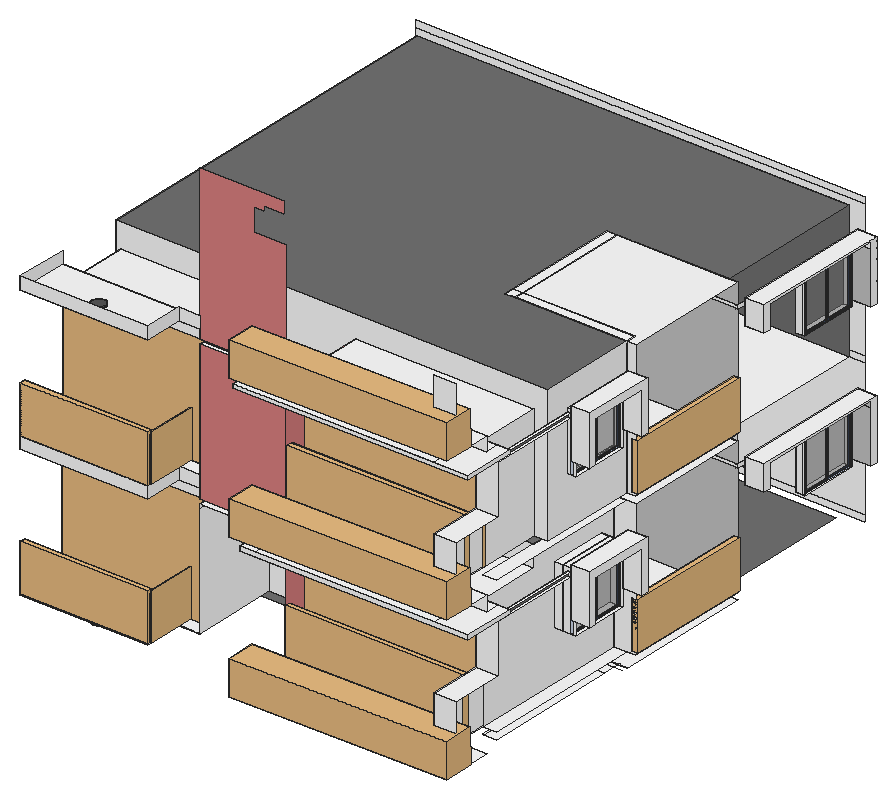
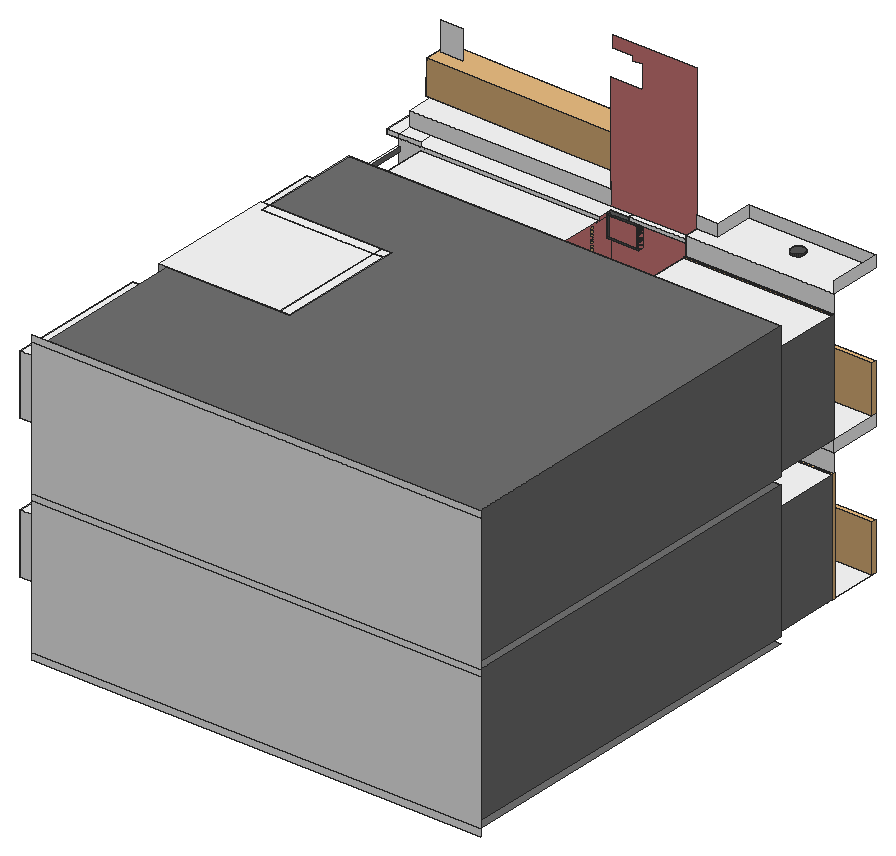
# SketchUp Ruby script. Lengths in inches.
U = 1.inch
M = Sketchup.active_model
def pt(a) = Geom::Point3d.new(a.map { |v| v * U })
def face(e, loops, mat)
  f = e.add_face(loops[0].map { |a| pt(a) })
  loops[1..].each { |l| e.add_face(l.map { |a| pt(a) }).erase! }
  f.material = f.back_material = mat if mat
  f
end
# faces: each face lists its corners as indices into pts; further lists are holes
def faces(e, pts, list, mat = nil) = list.each { |f| face(e, (f[0].is_a?(Array) ? f : [f]).map { |l| l.map { |i| pts[i] } }, mat) }
# xy, xz, yz: faces in a plane at the given z, y or x. An outline is a flat list of corners, or four numbers for a rectangle; further outlines are holes
def ring(l) = l.size == 4 ? [[l[0], l[1]], [l[2], l[1]], [l[2], l[3]], [l[0], l[3]]] : l.each_slice(2).to_a
def flat(e, list, mat, &to3) = list.each { |f| face(e, (f[0].is_a?(Array) ? f : [f]).map { |l| ring(l).map { |u, v| to3.(u, v) } }, mat) }
def xy(e, z, list, mat = nil) = flat(e, list, mat) { |x, y| [x, y, z] }
def xz(e, y, list, mat = nil) = flat(e, list, mat) { |x, z| [x, y, z] }
def yz(e, x, list, mat = nil) = flat(e, list, mat) { |y, z| [x, y, z] }
def lines(e, pts, list) = list.each { |a, b| e.add_line(pt(pts[a]), pt(pts[b])) }
# prism: a flat outline (further loops are holes) pulled along v
def prism(e, loops, v, mat = nil)
  f = face(e, loops, mat); d = Geom::Vector3d.new(v.map { |x| x * U })
  f.pushpull(f.normal.samedirection?(d) ? d.length : -d.length)
end
def box(e, o, s, mat = nil) = prism(e, [[o, [o[0] + s[0], o[1], o[2]], [o[0] + s[0], o[1] + s[1], o[2]], [o[0], o[1] + s[1], o[2]]]], [0, 0, s[2]], mat)
def at(x, y, z, deg = 0) = Geom::Transformation.translation(pt([x, y, z])) * Geom::Transformation.rotation(ORIGIN, Z_AXIS, deg.degrees)
def axes(o, x, y, z) = Geom::Transformation.new([*x, 0, *y, 0, *z, 0, *pt(o).to_a, 1])
def part(name) = M.definitions.add(name)
# library, detail: a bought-in or finely detailed component or shape, given as its bounding box
def library(name, o, s) = part(name).tap { |d| box(d.entities, o, s) }
def detail(e, o, s) = box(e.add_group.entities, o, s)
def put(e, d, t, mat = nil) = e.add_instance(d, t).tap { |i| i.material = mat if mat }
def group(e, t, mat = nil) = e.add_group.tap { |g| g.transformation = t; g.material = mat if mat }.entities
root = M.entities
M.materials.add("[Color M00]").color = [255, 255, 255]
M.materials.add("[Color M02]").color = [198, 198, 198]
M.materials.add("[Color M05]").color = [114, 114, 114]
M.materials.add("[Color M06]").color = [86, 86, 86]
M.materials.add("[Color_006]").color = [86, 86, 86]
M.materials.add("[Tile Various Tan]").color = [221, 130, 130]
M.materials.add("[Translucent Glass Blue]").color = [74, 111, 178]
M.materials["[Translucent Glass Blue]"].alpha = 0.26
M.materials.add("[Translucent Glass Gray]").color = [128, 128, 128]
M.materials["[Translucent Glass Gray]"].alpha = 0.5
M.materials.add("[Translucent_Glass_Gray]").color = [167, 187, 214]
M.materials["[Translucent_Glass_Gray]"].alpha = 0.8
c1 = library("Living wall panel",[-0.54,-4.26,-5.13],[55.52,26.12,125.59])
c2 = library("Glass Railing",[0,0,0],[139.5,4.76,42])
c3 = library("Glazed balcony doors",[0,0,0],[135.86,2.83,115.35])
c4 = part("glass-railing")
detail(c4.entities,[0,0,0],[1.26,75.59,33.1875])
c5 = part("Group\#3")
xy(c5.entities,0,[[0,0,32.48,1.97]])
xy(c5.entities,0.98,[[0.98,0,31.5,0.98],[0.98,0.98,31.5,1.97]])
xy(c5.entities,8.86,[[0.98,0,31.5,0.98],[0.98,0.98,31.5,1.97]])
xy(c5.entities,9.84,[[0,0,32.48,1.97]])
xz(c5.entities,0,[[[0,0,32.48,9.84],[0.98,0.98,31.5,8.86]]])
xz(c5.entities,0.98,[[0.98,0.98,31.5,8.86]],"[Translucent Glass Gray]")
xz(c5.entities,1.97,[[[0,0,32.48,9.84],[0.98,0.98,31.5,8.86]]])
yz(c5.entities,0,[[0,0,1.97,9.84]])
yz(c5.entities,0.98,[[0,0.98,0.98,8.86],[0.98,0.98,1.97,8.86]])
yz(c5.entities,31.5,[[0,0.98,0.98,8.86],[0.98,0.98,1.97,8.86]])
yz(c5.entities,32.48,[[0,0,1.97,9.84]])
c6 = part("Group\#4")
xy(c6.entities,0,[[0,0,32.48,1.97]])
xy(c6.entities,0.98,[[0.98,0,31.5,0.98],[0.98,0.98,31.5,1.97]])
xy(c6.entities,71.85,[[0.98,0,31.5,0.98],[0.98,0.98,31.5,1.97]])
xy(c6.entities,72.83,[[0,0,32.48,1.97]])
xz(c6.entities,0,[[[0,0,32.48,72.83],[0.98,0.98,31.5,71.85]]])
xz(c6.entities,0.98,[[0.98,0.98,31.5,71.85]],"[Translucent Glass Gray]")
xz(c6.entities,1.97,[[[0,0,32.48,72.83],[0.98,0.98,31.5,71.85]]])
yz(c6.entities,0,[[0,0,1.97,72.83]])
yz(c6.entities,0.98,[[0,0.98,0.98,71.85],[0.98,0.98,1.97,71.85]])
yz(c6.entities,31.5,[[0,0.98,0.98,71.85],[0.98,0.98,1.97,71.85]])
yz(c6.entities,32.48,[[0,0,1.97,72.83]])
c7 = part("Fixed transom window")
xy(c7.entities,0,[[0,0,70.86,3.9375]])
xy(c7.entities,1.97,[[1.97,0,34.45,0.98],[36.42,0,68.9,3.9375],[1.97,2.95,34.45,3.9375]])
xy(c7.entities,86.61,[[1.97,0,34.45,3.9375],[34.45,0,36.42,3.9375],[36.42,0,68.9,3.9375]])
xy(c7.entities,88.58,[[0,0,70.86,3.9375]])
xz(c7.entities,0,[[[0,0,70.86,88.58],[1.97,1.97,34.45,86.61],[36.42,1.97,68.9,86.61]]])
xz(c7.entities,3.9375,[[[0,0,70.86,88.58],[1.97,1.97,34.45,86.61],[36.42,1.97,68.9,86.61]]])
yz(c7.entities,0,[[0,0,3.9375,88.58]])
yz(c7.entities,1.97,[[0,1.97,3.9375,74.8],[0,76.77,3.9375,86.61]])
yz(c7.entities,34.45,[[0,1.97,3.9375,86.61]])
yz(c7.entities,36.42,[[0,1.97,3.9375,86.61]])
yz(c7.entities,68.9,[[0,1.97,3.9375,86.61]])
yz(c7.entities,70.86,[[0,0,3.9375,88.58]])
g1 = group(c7.entities,at(1.97,0,74.8))
box(g1,[0,0,0],[66.93,3.9375,1.97])
put(c7.entities,c5,at(1.97,0.98,76.77),"[Translucent Glass Blue]")
put(c7.entities,c5,at(36.42,0.98,76.77),"[Translucent Glass Blue]")
put(c7.entities,c6,at(1.97,0.98,1.97),"[Translucent Glass Blue]")
put(c7.entities,c6,at(36.42,0.98,1.97),"[Translucent Glass Blue]")
c8 = part("FIXED+GLASS+WINDOW+WITH+TRANSOM")
put(c8.entities,c7,at(0,0,0),"[Translucent Glass Blue]")
c9 = part("BIC_Bike Shop - Window - Small")
xy(c9.entities,-8,[[[0,0,36,36],[2,2,34,34]]],"[Color_006]")
xy(c9.entities,-4,[[2,2,34,34]],"[Translucent_Glass_Gray]")
xy(c9.entities,0,[[[0,0,36,36],[2,2,34,34]]],"[Color_006]")
xz(c9.entities,0,[[0,-8,36,0]],"[Color_006]")
xz(c9.entities,2,[[2,-8,34,-4],[2,-4,34,0]],"[Color_006]")
xz(c9.entities,34,[[2,-8,34,-4],[2,-4,34,0]],"[Color_006]")
xz(c9.entities,36,[[0,-8,36,0]],"[Color_006]")
yz(c9.entities,0,[[0,-8,36,0]],"[Color_006]")
yz(c9.entities,2,[[2,-8,34,-4],[2,-4,34,0]],"[Color_006]")
yz(c9.entities,34,[[2,-8,34,-4],[2,-4,34,0]],"[Color_006]")
yz(c9.entities,36,[[0,-8,36,0]],"[Color_006]")
xy(root,374.8125,[[129.49,93.91,127.93,94.12,126.49,94.72,125.24,95.67,124.29,96.91,123.69,98.36,123.49,99.91,123.69,101.46,124.29,102.91,125.24,104.15,126.49,105.11,127.93,105.71,129.49,105.91,131.04,105.71,132.49,105.11,133.73,104.15,134.68,102.91,135.28,101.46,135.49,99.91,135.28,98.36,134.68,96.91,133.73,95.67,132.49,94.72,131.04,94.12]],"[Color M06]")
xy(root,377.5625,[[281.18,83.25,458.625,117.625],[439.42,137.58,439.8125,257.51],[439.8125,137.58,450.92,257.51],[330.6875,194.2,330.6875,281.78,385.6875,281.78,385.6875,273.63,401.8125,273.63,401.8125,257.51,439.42,257.51,439.42,194.2],[401.8125,257.51,439.42,267.63],
  [439.42,257.51,450.92,267.63],[401.8125,267.63,439.42,272.07],[439.42,267.63,450.92,272.07],[401.8125,272.07,439.42,273.63],[439.42,272.07,450.92,273.63],
  [450.92,272.07,458.625,273.63],[385.6875,273.63,401.8125,281.78],[401.8125,273.63,458.625,394.46],[385.6875,281.78,401.8125,394.46]],"[Color M00]")
xy(root,377.5625,[[69.2,194.2,69.2,527.42,439.42,527.42,439.42,394.46,385.6875,394.46,385.6875,281.78,330.6875,281.78,330.6875,194.2]],"[Color M05]")
xy(root,383.5625,[[73.74,83.25,73.74,137.58,204.98,137.58,204.98,117.625,186.35,117.625,186.35,83.25],[281.18,91.3,439.11,137.58],[73.74,137.58,204.98,137.58,204.98,194.2,281.18,194.2,281.18,137.58,439.11,137.58,439.11,281.78,351.1875,281.78,351.1875,527.42,69.2,527.42,69.2,194.2,73.74,194.2],[439.11,137.58,450.92,281.78],[351.1875,281.78,439.11,290.48],
  [439.11,281.78,450.92,281.78,450.92,394.46,351.1875,394.46,351.1875,290.48,439.11,290.48],[450.92,281.78,458.625,394.46]],"[Color M00]")
xy(root,383.8125,[[73.74,83.25,186.35,83.25,186.35,117.625,204.98,117.625,204.98,137.58,73.74,137.58],[281.18,91.3,439.11,137.58]],"[Color M00]")
xy(root,397,[[281.18,83.25,439.11,91.3]],"[Color M00]")
xy(root,397.25,[[281.18,83.25,439.11,91.3]],"[Color M00]")
xy(root,427.98,[[438.17,215.57,446.875,267.63],[446.875,215.57,458.625,267.63],[450.92,468.92,458.625,520.98]],"[Color M00]")
xy(root,433.84,[[439.11,83.25,458.625,129.875]],"[Color M00]")
xy(root,434.24,[[458.625,520.98,475.1875,526.98]],"[Color M00]")
xy(root,442.95,[[458.625,210.07,475.5625,215.57],[458.625,267.63,475.5625,273.63]],"[Color M00]")
xy(root,465.36,[[458.625,402.98,475.1875,408.98]],"[Color M00]")
xy(root,466.54,[[252.64,117.625,281.18,122.0625]],"[Tile Various Tan]")
xy(root,477.21,[[456.375,130.82,458.625,210.07]],"[Color M00]")
xy(root,480.05,[[438.17,215.57,446.875,267.63],[446.875,215.57,458.625,267.63],[458.625,215.57,475.5625,267.63],[450.92,468.92,458.625,520.98]],"[Color M00]")
xy(root,481.21,[[456.375,130.82,458.625,210.07]],"[Color M00]")
xy(root,482.19,[[381.625,394.46,385.6875,394.83],[385.6875,394.46,401.8125,394.83],[401.8125,394.46,458.625,394.83]],"[Color M00]")
xy(root,482.48,[[73.74,129.875,204.98,194.2]],"[Color M00]")
xy(root,484.125,[[281.18,129.875,439.11,194.2]],"[Color M00]")
xy(root,485.48,[[381.625,394.46,385.6875,394.83],[385.6875,394.46,401.8125,394.83],[401.8125,394.46,458.625,394.83],[458.625,394.46,459,400.46]],"[Color M00]")
xy(root,485.49,[[458.625,408.98,475.1875,520.98]],"[Color M00]")
xy(root,486.52,[[267.54,83.25,267.54,122.0625,281.18,122.0625,281.18,129.875,468.99,129.875,468.99,83.25],[204.98,117.625,252.64,117.625,252.64,122.0625,267.54,122.0625,267.54,123.3125,204.98,123.3125]],"[Color M00]")
xy(root,486.64,[[458.625,210.07,475.5625,273.63]],"[Color M00]")
xy(root,487.3,[[458.625,402.98,475.1875,526.98]],"[Color M00]")
xy(root,490.2,[[267.54,83.25,281.18,117.625],[281.18,83.25,439.24,117.625],[439.24,83.25,468.99,83.25,468.99,129.875,458.625,129.875,458.625,117.625,439.24,117.625],[204.98,117.625,267.54,123.3125],[439.24,117.625,458.625,129.875]],"[Color M00]")
xy(root,498.9375,[[[73.74,83.25,73.74,129.875,204.98,129.875,204.98,117.625,186.35,117.625,186.35,83.25],[129.49,93.91,131.04,94.12,132.49,94.72,133.73,95.67,134.68,96.91,135.28,98.36,135.49,99.91,135.28,101.46,134.68,102.91,133.73,104.15,132.49,105.11,131.04,105.71,129.49,105.91,127.93,105.71,126.49,105.11,125.24,104.15,124.29,102.91,123.69,101.46,123.49,99.91,123.69,98.36,124.29,96.91,125.24,95.67,126.49,94.72,127.93,94.12]]],"[Color M00]")
xy(root,500.8125,[[129.49,93.91,127.93,94.12,126.49,94.72,125.24,95.67,124.29,96.91,123.69,98.36,123.49,99.91,123.69,101.46,124.29,102.91,125.24,104.15,126.49,105.11,127.93,105.71,129.49,105.91,131.04,105.71,132.49,105.11,133.73,104.15,134.68,102.91,135.28,101.46,135.49,99.91,135.28,98.36,134.68,96.91,133.73,95.67,132.49,94.72,131.04,94.12]],"[Color M06]")
xy(root,503.5625,[[281.18,83.25,458.625,117.625],[439.11,137.58,450.92,281.78],[351.1875,281.78,439.11,290.48],[439.11,281.78,439.11,290.48,351.1875,290.48,351.1875,394.46,458.625,394.46,458.625,281.78]],"[Color M00]")
xy(root,503.5625,[[69.2,194.2,69.2,527.42,351.1875,527.42,351.1875,281.78,439.11,281.78,439.11,194.2]],"[Color M05]")
xy(root,509.5625,[[73.74,83.25,186.35,83.25,186.35,117.625,204.98,117.625,204.98,129.875,73.74,129.875],[281.18,91.3,439.11,137.58],[73.74,129.875,204.98,137.58],[73.74,137.58,204.98,137.58,204.98,194.2,281.18,194.2,281.18,137.58,343.48,137.58,343.48,394.46,450.92,394.46,450.92,527.42,69.2,527.42,69.2,194.2,73.74,194.2],[343.48,137.58,439.11,137.58,439.11,194.2,450.92,194.2,450.92,281.78,343.48,281.78],
  [343.48,281.78,352.1875,290.48],[352.1875,281.78,450.92,290.48],[450.92,281.78,458.625,394.46],[343.48,290.48,352.1875,394.46],[352.1875,290.48,450.92,394.46]],"[Color M00]")
xy(root,509.8125,[[281.18,91.3,439.11,137.58],[73.74,129.875,204.98,137.58]],"[Color M00]")
xy(root,523,[[281.18,83.25,439.11,91.3]],"[Color M00]")
xy(root,523.25,[[281.18,83.25,439.11,91.3]],"[Color M00]")
xy(root,553.98,[[450.92,215.57,458.625,267.63],[450.92,468.92,458.625,520.98]],"[Color M00]")
xy(root,559.84,[[439.11,83.25,458.625,129.875]],"[Color M00]")
xy(root,560.24,[[458.625,520.98,475.1875,526.98]],"[Color M00]")
xy(root,568.95,[[458.625,210.07,475.5625,215.57],[458.625,267.63,475.5625,273.63]],"[Color M00]")
xy(root,591.36,[[458.625,402.98,475.1875,408.98]],"[Color M00]")
xy(root,592.97,[[252.64,117.625,281.18,121.75]],"[Tile Various Tan]")
xy(root,603.27,[[456.375,130.82,458.625,210.07]],"[Color M00]")
xy(root,606.05,[[450.92,215.57,458.625,267.63],[458.625,215.57,475.5625,267.63],[450.92,468.92,458.625,520.98]],"[Color M00]")
xy(root,607.27,[[456.375,130.82,458.625,210.07]],"[Color M00]")
xy(root,608.19,[[381.625,394.46,385.6875,394.83],[385.6875,394.46,401.8125,394.83],[401.8125,394.46,458.625,394.83]],"[Color M00]")
xy(root,608.48,[[73.74,129.875,204.98,194.2]],"[Color M00]")
xy(root,610.125,[[281.18,129.875,439.11,194.2]],"[Color M00]")
xy(root,611.48,[[381.625,394.46,385.6875,394.83],[385.6875,394.46,401.8125,394.83],[401.8125,394.46,458.625,394.83],[458.625,394.46,459,400.46]],"[Color M00]")
xy(root,611.49,[[458.625,408.98,475.1875,520.98]],"[Color M00]")
xy(root,612.64,[[458.625,210.07,475.5625,273.63]],"[Color M00]")
xy(root,612.95,[[261.54,83.25,261.54,121.75,281.18,121.75,281.18,129.875,468.99,129.875,468.99,83.25],[204.98,117.625,252.64,121.75]],"[Color M00]")
xy(root,613.3,[[458.625,402.98,475.1875,526.98]],"[Color M00]")
xy(root,616.64,[[261.54,83.25,439.24,117.625],[439.24,83.25,468.99,83.25,468.99,129.875,458.625,129.875,458.625,117.625,439.24,117.625],[204.98,117.625,261.54,121.75],[439.24,117.625,458.625,129.875]],"[Color M00]")
xy(root,624.9375,[[[73.74,83.25,73.74,129.875,204.98,129.875,204.98,117.625,186.35,117.625,186.35,83.25],[129.49,93.91,131.04,94.12,132.49,94.72,133.73,95.67,134.68,96.91,135.28,98.36,135.49,99.91,135.28,101.46,134.68,102.91,133.73,104.15,132.49,105.11,131.04,105.71,129.49,105.91,127.93,105.71,126.49,105.11,125.24,104.15,124.29,102.91,123.69,101.46,123.49,99.91,123.69,98.36,124.29,96.91,125.24,95.67,126.49,94.72,127.93,94.12]]],"[Color M00]")
xy(root,626.8125,[[129.49,93.91,127.93,94.12,126.49,94.72,125.24,95.67,124.29,96.91,123.69,98.36,123.49,99.91,123.69,101.46,124.29,102.91,125.24,104.15,126.49,105.11,127.93,105.71,129.49,105.91,131.04,105.71,132.49,105.11,133.73,104.15,134.68,102.91,135.28,101.46,135.49,99.91,135.28,98.36,134.68,96.91,133.73,95.67,132.49,94.72,131.04,94.12]],"[Color M06]")
xy(root,629.5625,[[281.18,83.25,458.625,117.625],[343.48,281.78,352.1875,290.48],[352.1875,281.78,450.92,290.48],[450.92,281.78,450.92,290.48,352.1875,290.48,352.1875,394.46,458.625,394.46,458.625,281.78],[343.48,290.48,352.1875,394.46]],"[Color M00]")
xy(root,629.5625,[[69.2,194.2,69.2,527.42,450.92,527.42,450.92,394.46,343.48,394.46,343.48,281.78,450.92,281.78,450.92,194.2]],"[Color M05]")
xz(root,83.25,[[281.18,377.5625,458.625,377.5625,458.625,433.84,439.11,433.84,439.11,397,281.18,397],[73.74,383.5625,186.35,383.8125],[281.18,397,439.11,397.25],[267.54,486.52,468.99,490.2],[73.74,498.9375,186.35,509.5625],
  [281.18,503.5625,458.625,503.5625,458.625,559.84,439.11,559.84,439.11,523,281.18,523],[281.18,523,439.11,523.25],[261.54,612.95,468.99,616.64],[73.74,624.9375,186.35,635.5625],[281.18,629.5625,458.625,629.5625,458.625,685.84,439.11,685.84,439.11,649,281.18,649]],"[Color M00]")
xz(root,91.3,[[281.18,383.5625,439.11,383.8125],[281.18,383.8125,439.11,397],[281.18,397,439.11,397.25],[281.18,509.5625,439.11,509.8125],[281.18,509.8125,439.11,523],
  [281.18,523,439.11,523.25]],"[Color M00]")
xz(root,117.625,[[186.35,383.5625,204.98,383.8125],[281.18,490.2,458.625,503.5625],[186.35,498.9375,204.98,509.5625],[281.18,616.64,458.625,629.5625],[186.35,624.9375,204.98,635.5625]],"[Color M00]")
xz(root,117.625,[[204.98,490.2,281.18,490.2,281.18,592.97,252.64,592.97,252.64,612.95,204.98,612.95],[204.98,616.64,281.18,616.64,281.18,718.41,252.64,718.41,252.64,738.39,261.54,738.39,261.54,742.08,279.24,742.08,279.24,752.39,204.98,752.39]],"[Tile Various Tan]")
xz(root,121.75,[[204.98,612.95,261.54,616.64]],"[Color M00]")
xz(root,121.75,[[252.64,592.97,281.18,612.95]],"[Tile Various Tan]")
xz(root,122.0625,[[252.64,466.54,281.18,486.52]],"[Tile Various Tan]")
xz(root,123.3125,[[204.98,486.52,267.54,490.2]],"[Color M00]")
xz(root,129.875,[[439.11,433.84,458.625,433.84,458.625,486.52,281.18,486.52,281.18,484.125,439.11,484.125],[73.74,482.48,204.98,498.9375],[439.24,486.52,458.625,490.2],[458.625,486.52,468.99,490.2],[73.74,498.9375,204.98,509.5625],
  [73.74,509.5625,204.98,509.8125],[439.11,559.84,458.625,559.84,458.625,612.95,281.18,612.95,281.18,610.125,439.11,610.125],[73.74,608.48,204.98,624.9375],[439.24,612.95,458.625,616.64],[458.625,612.95,468.99,616.64]],"[Color M00]")
xz(root,130.82,[[456.375,477.21,458.625,481.21],[456.375,603.27,458.625,607.27]],"[Color M00]")
xz(root,137.58,[[73.74,383.5625,204.98,383.8125],[281.18,383.5625,439.11,383.8125],[73.74,509.5625,204.98,509.8125],[281.18,509.5625,343.48,509.8125],[343.48,509.5625,439.11,509.8125]],"[Color M00]")
xz(root,194.2,[[69.2,383.5625,69.2,503.5625,439.11,503.5625,439.11,484.125,281.18,484.125,281.18,383.5625,204.98,383.5625,204.98,482.48,73.74,482.48,73.74,383.5625],[69.2,509.5625,69.2,629.5625,450.92,629.5625,450.92,509.5625,439.11,509.5625,439.11,610.125,281.18,610.125,281.18,509.5625,204.98,509.5625,204.98,608.48,73.74,608.48,73.74,509.5625]],"[Color M00]")
xz(root,210.07,[[458.625,442.95,475.5625,486.64],[456.375,477.21,458.625,480.05],[456.375,480.05,458.625,481.21],[458.625,568.95,475.5625,612.64],[456.375,603.27,458.625,606.11],
  [456.375,606.11,458.625,607.27]],"[Color M00]")
xz(root,215.57,[[438.17,427.98,446.875,480.05],[446.875,427.98,458.625,480.05],[458.625,442.95,475.5625,480.05],[450.92,553.98,458.625,606.05],[458.625,568.95,475.5625,606.05]],"[Color M00]")
xz(root,267.63,[[438.17,427.98,446.875,480.05],[446.875,427.98,458.625,480.05],[458.625,442.95,475.5625,480.05],[450.92,553.98,458.625,606.05],[458.625,568.95,475.5625,606.05]],"[Color M00]")
xz(root,273.63,[[458.625,442.95,475.5625,486.64],[458.625,568.95,475.5625,612.64]],"[Color M00]")
xz(root,281.78,[[351.1875,383.5625,439.11,503.5625],[439.11,383.5625,458.625,503.5625],[343.48,509.5625,352.1875,629.5625],[352.1875,509.5625,450.92,629.5625],[450.92,509.5625,458.625,629.5625]],"[Color M00]")
xz(root,290.48,[[351.1875,383.5625,439.11,503.5625],[343.48,509.5625,352.1875,629.5625],[352.1875,509.5625,450.92,629.5625]],"[Color M00]")
xz(root,394.46,[[343.48,509.5625,352.1875,629.5625]],"[Color M00]")
xz(root,394.46,[[351.1875,383.5625,458.625,383.5625,458.625,482.19,381.625,482.19,381.625,485.48,458.625,485.48,458.625,503.5625,351.1875,503.5625],[352.1875,509.5625,458.625,509.5625,458.625,608.19,381.625,608.19,381.625,611.48,458.625,611.48,458.625,629.5625,352.1875,629.5625]],"[Color M02]")
xz(root,394.83,[[381.625,482.19,458.625,485.48],[381.625,608.19,458.625,611.48]],"[Color M00]")
xz(root,400.46,[[458.625,482.11,459,485.48],[458.625,608.11,459,611.48]],"[Color M00]")
xz(root,402.98,[[458.625,465.36,475.1875,487.3],[458.625,591.36,475.1875,613.3]],"[Color M00]")
xz(root,408.98,[[458.625,465.36,475.1875,479.49],[458.625,479.49,475.1875,485.49],[458.625,591.36,475.1875,605.49],[458.625,605.49,475.1875,611.49]],"[Color M00]")
xz(root,468.92,[[450.92,427.98,458.625,480.05],[450.92,553.98,458.625,606.05]],"[Color M00]")
xz(root,520.98,[[450.92,427.98,458.625,480.05],[450.92,553.98,458.625,606.05],[458.625,606.05,475.1875,611.49]],"[Color M00]")
xz(root,520.98,[[458.625,434.24,475.1875,480.05],[458.625,480.05,475.1875,485.49],[458.625,560.24,475.1875,606.05]],"[Color M02]")
xz(root,526.98,[[458.625,434.24,475.1875,487.3],[458.625,560.24,475.1875,613.3]],"[Color M00]")
xz(root,527.42,[[69.2,383.5625,351.1875,503.5625],[69.2,509.5625,450.92,629.5625]],"[Color M05]")
xz(root,535.125,[[61.5,377.5625,458.625,383.5625],[61.5,383.5625,458.625,503.5625],[61.5,503.5625,458.625,509.5625],[61.5,509.5625,458.625,629.5625],[61.5,629.5625,458.625,635.5625]],"[Color M00]")
yz(root,69.2,[[194.2,383.5625,527.42,503.5625],[194.2,509.5625,527.42,629.5625]],"[Color M05]")
yz(root,73.74,[[83.25,383.5625,129.875,383.8125],[129.875,383.5625,137.58,383.8125],[83.25,498.9375,129.875,509.5625],[129.875,509.5625,137.58,509.8125],[83.25,624.9375,129.875,635.5625]],"[Color M00]")
yz(root,73.74,[[137.58,383.5625,194.2,383.5625,194.2,482.48,129.875,482.48,129.875,383.8125,137.58,383.8125],[137.58,509.5625,194.2,509.5625,194.2,608.48,129.875,608.48,129.875,509.8125,137.58,509.8125]],"[Color M05]")
yz(root,186.35,[[83.25,383.5625,117.625,383.8125],[83.25,498.9375,117.625,509.5625],[83.25,624.9375,117.625,635.5625]],"[Color M00]")
yz(root,204.98,[[117.625,383.5625,137.58,383.8125],[137.58,383.5625,137.58,383.8125,117.625,383.8125,117.625,482.48,194.2,482.48,194.2,383.5625],[117.625,482.48,117.625,486.52,123.3125,486.52,123.3125,490.2,117.625,490.2,117.625,498.9375,129.875,498.9375,129.875,482.48],[117.625,498.9375,129.875,509.5625],[117.625,509.5625,117.625,608.48,194.2,608.48,194.2,509.5625,137.58,509.5625,137.58,509.8125,129.875,509.8125,129.875,509.5625],
  [129.875,509.5625,137.58,509.8125],[117.625,608.48,117.625,612.95,121.75,612.95,121.75,616.64,117.625,616.64,117.625,624.9375,129.875,624.9375,129.875,608.48]],"[Color M00]")
yz(root,252.64,[[117.625,466.54,122.0625,486.52],[117.625,592.97,121.75,612.95]],"[Tile Various Tan]")
yz(root,261.54,[[83.25,612.95,121.75,616.64]],"[Color M00]")
yz(root,267.54,[[83.25,486.52,123.3125,490.2]],"[Color M00]")
yz(root,281.18,[[83.25,377.5625,83.25,397,91.3,397,91.3,383.5625,117.625,383.5625,117.625,377.5625],[91.3,383.5625,117.625,383.8125],[117.625,383.5625,137.58,383.8125],[83.25,397,91.3,397.25],[83.25,503.5625,83.25,523,91.3,523,91.3,509.5625,117.625,509.5625,117.625,503.5625],
  [91.3,509.5625,117.625,509.8125],[117.625,509.5625,137.58,509.8125],[83.25,523,91.3,523.25],[83.25,629.5625,83.25,649,91.3,649,91.3,635.5625,117.625,635.5625,117.625,629.5625]],"[Color M00]")
yz(root,281.18,[[137.58,383.5625,194.2,383.5625,194.2,484.125,122.0625,484.125,122.0625,466.54,117.625,466.54,117.625,383.8125,137.58,383.8125],[122.0625,484.125,129.875,486.52],[137.58,509.5625,194.2,509.5625,194.2,610.125,121.75,610.125,121.75,592.97,117.625,592.97,117.625,509.8125,137.58,509.8125],[121.75,610.125,129.875,612.95]],"[Tile Various Tan]")
yz(root,343.48,[[281.78,509.5625,290.48,629.5625],[290.48,509.5625,394.46,629.5625]],"[Color M00]")
yz(root,351.1875,[[281.78,383.5625,290.48,503.5625],[290.48,383.5625,394.46,503.5625],[394.46,383.5625,527.42,503.5625]],"[Color M00]")
yz(root,352.1875,[[281.78,509.5625,290.48,629.5625],[290.48,509.5625,394.46,629.5625]],"[Color M00]")
yz(root,381.625,[[394.46,482.19,394.83,485.48],[394.46,608.19,394.83,611.48]],"[Color M00]")
yz(root,438.17,[[215.57,427.98,267.63,480.05]],"[Color M00]")
yz(root,439.11,[[91.3,383.5625,137.58,383.8125],[137.58,383.5625,137.58,484.125,194.2,484.125,194.2,503.5625,281.78,503.5625,281.78,383.5625],[281.78,383.5625,290.48,503.5625],[91.3,383.8125,91.3,397.25,83.25,397.25,83.25,433.84,129.875,433.84,129.875,484.125,137.58,484.125,137.58,383.8125],[83.25,397,91.3,397.25],
  [137.58,509.5625,137.58,509.8125,91.3,509.8125,91.3,523.25,83.25,523.25,83.25,559.84,129.875,559.84,129.875,610.125,194.2,610.125,194.2,509.5625],[91.3,509.5625,137.58,509.8125],[83.25,523,91.3,523.25]],"[Color M00]")
yz(root,446.875,[[215.57,427.98,267.63,480.05]],"[Color M00]")
yz(root,450.92,[[468.92,427.98,520.98,480.05],[[194.2,509.5625,281.78,629.5625],[215.57,553.98,267.63,606.05]],[281.78,509.5625,290.48,629.5625]],"[Color M00]")
yz(root,456.375,[[130.82,477.21,210.07,481.21],[130.82,603.27,210.07,607.27]],"[Color M05]")
yz(root,458.625,[[520.98,434.24,520.98,485.49,408.98,485.49,408.98,465.36,402.98,465.36,402.98,487.3,526.98,487.3,526.98,434.24],[210.07,442.95,210.07,486.64,273.63,486.64,273.63,442.95,267.63,442.95,267.63,480.05,215.57,480.05,215.57,442.95],[394.46,482.19,394.83,485.48],[520.98,560.24,520.98,611.49,408.98,611.49,408.98,591.36,402.98,591.36,402.98,613.3,526.98,613.3,526.98,560.24],[210.07,568.95,210.07,612.64,273.63,612.64,273.63,568.95,267.63,568.95,267.63,606.05,215.57,606.05,215.57,568.95],
  [394.46,608.19,394.83,611.48]],"[Color M00]")
yz(root,459,[[400.46,482.11,400.46,485.48,394.46,485.48,394.46,482.19],[400.46,608.11,400.46,611.48,394.46,611.48,394.46,608.19]],"[Color M00]")
yz(root,468.99,[[83.25,486.52,129.875,490.2],[83.25,612.95,129.875,616.64]],"[Color M00]")
yz(root,475.1875,[[520.98,434.24,526.98,434.24,526.98,487.3,402.98,487.3,402.98,465.36,408.98,465.36,408.98,485.49,520.98,485.49],[520.98,560.24,526.98,560.24,526.98,613.3,402.98,613.3,402.98,591.36,408.98,591.36,408.98,611.49,520.98,611.49]],"[Color M00]")
yz(root,475.5625,[[210.07,442.95,215.57,442.95,215.57,480.05,267.63,480.05,267.63,442.95,273.63,442.95,273.63,486.64,210.07,486.64],[210.07,568.95,215.57,568.95,215.57,606.05,267.63,606.05,267.63,568.95,273.63,568.95,273.63,612.64,210.07,612.64]],"[Color M00]")
p = [[459,400.46,482.11],[459,394.46,482.19],[458.625,394.46,482.19],[458.625,400.46,482.11],[129.49,93.91,498.9375],[127.93,94.12,498.9375],
  [127.93,94.12,500.8125],[129.49,93.91,500.8125],[131.04,94.12,498.9375],[131.04,94.12,500.8125],[126.49,94.72,498.9375],[126.49,94.72,500.8125],
  [132.49,94.72,498.9375],[132.49,94.72,500.8125],[125.24,95.67,498.9375],[125.24,95.67,500.8125],[133.73,95.67,498.9375],[133.73,95.67,500.8125],
  [124.29,96.91,498.9375],[124.29,96.91,500.8125],[134.68,96.91,498.9375],[134.68,96.91,500.8125],[123.69,98.36,498.9375],[123.69,98.36,500.8125],
  [135.28,98.36,498.9375],[135.28,98.36,500.8125],[123.49,99.91,498.9375],[123.49,99.91,500.8125],[135.49,99.91,498.9375],[135.49,99.91,500.8125],
  [123.69,101.46,498.9375],[123.69,101.46,500.8125],[135.28,101.46,498.9375],[135.28,101.46,500.8125],[124.29,102.91,498.9375],[124.29,102.91,500.8125],
  [134.68,102.91,498.9375],[134.68,102.91,500.8125],[125.24,104.15,498.9375],[125.24,104.15,500.8125],[133.73,104.15,498.9375],[133.73,104.15,500.8125],
  [126.49,105.11,498.9375],[126.49,105.11,500.8125],[132.49,105.11,498.9375],[132.49,105.11,500.8125],[127.93,105.71,498.9375],[127.93,105.71,500.8125],
  [131.04,105.71,498.9375],[131.04,105.71,500.8125],[129.49,105.91,498.9375],[129.49,105.91,500.8125],[459,400.46,608.11],[459,394.46,608.19],
  [458.625,394.46,608.19],[458.625,400.46,608.11],[129.49,93.91,624.9375],[127.93,94.12,624.9375],[127.93,94.12,626.8125],[129.49,93.91,626.8125],
  [131.04,94.12,624.9375],[131.04,94.12,626.8125],[126.49,94.72,624.9375],[126.49,94.72,626.8125],[132.49,94.72,624.9375],[132.49,94.72,626.8125],
  [125.24,95.67,624.9375],[125.24,95.67,626.8125],[133.73,95.67,624.9375],[133.73,95.67,626.8125],[124.29,96.91,624.9375],[124.29,96.91,626.8125],
  [134.68,96.91,624.9375],[134.68,96.91,626.8125],[123.69,98.36,624.9375],[123.69,98.36,626.8125],[135.28,98.36,624.9375],[135.28,98.36,626.8125],
  [123.49,99.91,624.9375],[123.49,99.91,626.8125],[135.49,99.91,624.9375],[135.49,99.91,626.8125],[123.69,101.46,624.9375],[123.69,101.46,626.8125],
  [135.28,101.46,624.9375],[135.28,101.46,626.8125],[124.29,102.91,624.9375],[124.29,102.91,626.8125],[134.68,102.91,624.9375],[134.68,102.91,626.8125],
  [125.24,104.15,624.9375],[125.24,104.15,626.8125],[133.73,104.15,624.9375],[133.73,104.15,626.8125],[126.49,105.11,624.9375],[126.49,105.11,626.8125],
  [132.49,105.11,624.9375],[132.49,105.11,626.8125],[127.93,105.71,624.9375],[127.93,105.71,626.8125],[131.04,105.71,624.9375],[131.04,105.71,626.8125],
  [129.49,105.91,624.9375],[129.49,105.91,626.8125],[458.625,267.63,377.5625],[450.92,267.63,377.5625]]
faces(root,p,[[0,1,2,3],[52,53,54,55]],"[Color M00]")
faces(root,p,[[4,5,6,7],[8,4,7,9],[5,10,11,6],[12,8,9,13],[10,14,15,11],[16,12,13,17],[14,18,19,15],[20,16,17,21],
  [18,22,23,19],[24,20,21,25],[22,26,27,23],[28,24,25,29],[26,30,31,27],[32,28,29,33],[30,34,35,31],[36,32,33,37],
  [34,38,39,35],[40,36,37,41],[38,42,43,39],[44,40,41,45],[42,46,47,43],[48,44,45,49],[46,50,51,47],[50,48,49,51],
  [56,57,58,59],[60,56,59,61],[57,62,63,58],[64,60,61,65],[62,66,67,63],[68,64,65,69],[66,70,71,67],[72,68,69,73],
  [70,74,75,71],[76,72,73,77],[74,78,79,75],[80,76,77,81],[78,82,83,79],[84,80,81,85],[82,86,87,83],[88,84,85,89],
  [86,90,91,87],[92,88,89,93],[90,94,95,91],[96,92,93,97],[94,98,99,95],[100,96,97,101],[98,102,103,99],[102,100,101,103]],"[Color M06]")
lines(root,p,[[104,105]])
put(root,c1,axes([275.83,74.53,406.6875],[0.0058,0,-0.53997],[0,1,0],[1.53606,0,0.0165]),"[Color M00]")
put(root,c2,axes([281.18,115.6875,380.65],[1.13217,0,0],[0,1,0],[0,0,1.26661]),"[Color M00]")
put(root,c3,axes([73.4375,129.49,383.55],[0.96594,0,0],[0,0.86,0],[0,0,0.86]),"[Color M00]")
put(root,c3,axes([280.81,137.58,383.55],[1.16249,0,0],[0,0.86,0],[0,0,0.86]),"[Color M00]")
put(root,c2,axes([73.74,83.25,383.8125],[0.80723,0,0],[0,1,0],[0,0,1]),"[Color M00]")
put(root,c4,axes([186.35,85.95,383.9],[1,0,0],[0,1,0],[0,0,1.24195]),"[Color M00]")
put(root,c2,axes([460.38,281.78,385.99],[0,0.80723,0],[-1,0,0],[0,0,1]),"[Color M00]")
put(root,c8,axes([458.625,469.08,427.98],[0,0.73244,0],[-0.59,0,0],[0,0,0.57689]),"[Color M00]")
put(root,c8,axes([457.01,215.57,427.98],[0,0.73468,0],[-0.59,0,0],[0,0,0.59]),"[Color M00]")
put(root,c9,axes([252.64,117.625,466.54],[0.79273,0,0],[0,0,0.56],[0,-0.56,0]))
put(root,c1,axes([275.83,74.53,532.6875],[0.0058,0,-0.53997],[0,1,0],[1.53606,0,0.0165]),"[Color M00]")
put(root,c2,axes([73.74,83.25,509.5625],[0.80723,0,0],[0,1,0],[0,0,1]),"[Color M00]")
put(root,c2,axes([281.18,117.625,509.5625],[1.13217,0,0],[0,1,0],[0,0,1.19717]),"[Color M00]")
put(root,c4,axes([186.35,85.95,509.65],[1,0,0],[0,1,0],[0,0,1.24195]),"[Color M00]")
put(root,c3,axes([73.74,129.875,509.8125],[0.96594,0,0],[0,0.86,0],[0,0,0.86]),"[Color M00]")
put(root,c3,axes([281.18,136.9375,509.8125],[1.16249,0,0],[0,0.86,0],[0,0,0.86]),"[Color M00]")
put(root,c2,axes([460.38,281.78,511.99],[0,0.80723,0],[-1,0,0],[0,0,1]),"[Color M00]")
put(root,c8,axes([457.01,215.57,553.98],[0,0.73468,0],[-0.59,0,0],[0,0,0.59]),"[Color M00]")
put(root,c8,axes([458.625,469.08,553.98],[0,0.73244,0],[-0.59,0,0],[0,0,0.57689]),"[Color M00]")
put(root,c9,axes([252.64,117.625,592.97],[0.79273,0,0],[0,0,0.56],[0,-0.56,0]))
put(root,c1,axes([275.83,74.53,658.6875],[0.0058,0,-0.53997],[0,1,0],[1.53606,0,0.0165]),"[Color M00]")
